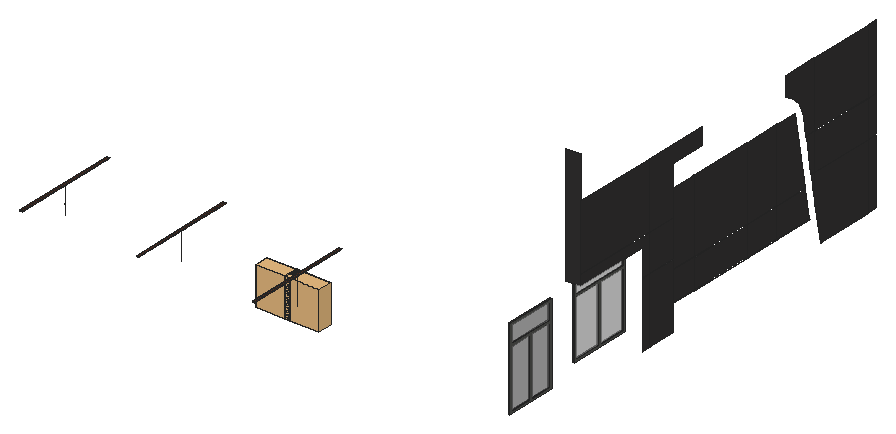
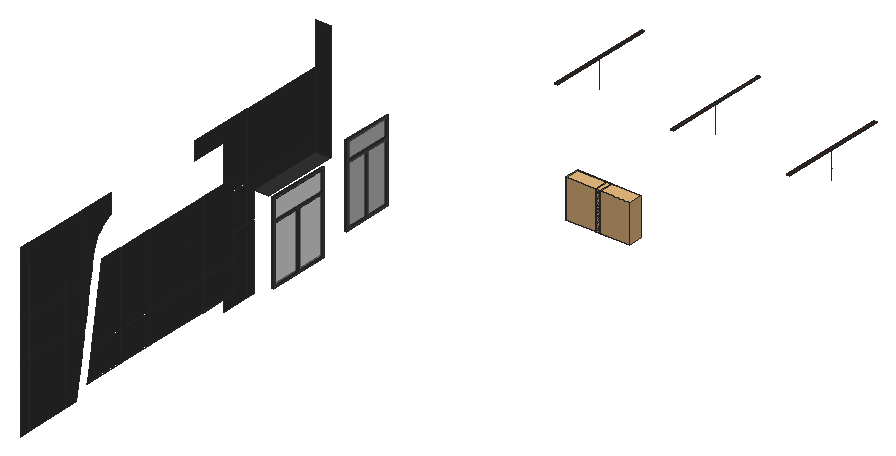
# SketchUp Ruby script. Lengths in inches.
U = 1.inch
M = Sketchup.active_model
def pt(a) = Geom::Point3d.new(a.map { |v| v * U })
def face(e, loops, mat)
  f = e.add_face(loops[0].map { |a| pt(a) })
  loops[1..].each { |l| e.add_face(l.map { |a| pt(a) }).erase! }
  f.material = f.back_material = mat if mat
  f
end
# faces: each face lists its corners as indices into pts; further lists are holes
def faces(e, pts, list, mat = nil) = list.each { |f| face(e, (f[0].is_a?(Array) ? f : [f]).map { |l| l.map { |i| pts[i] } }, mat) }
# xy, xz, yz: faces in a plane at the given z, y or x. An outline is a flat list of corners, or four numbers for a rectangle; further outlines are holes
def ring(l) = l.size == 4 ? [[l[0], l[1]], [l[2], l[1]], [l[2], l[3]], [l[0], l[3]]] : l.each_slice(2).to_a
def flat(e, list, mat, &to3) = list.each { |f| face(e, (f[0].is_a?(Array) ? f : [f]).map { |l| ring(l).map { |u, v| to3.(u, v) } }, mat) }
def xy(e, z, list, mat = nil) = flat(e, list, mat) { |x, y| [x, y, z] }
def xz(e, y, list, mat = nil) = flat(e, list, mat) { |x, z| [x, y, z] }
def yz(e, x, list, mat = nil) = flat(e, list, mat) { |y, z| [x, y, z] }
def lines(e, pts, list) = list.each { |a, b| e.add_line(pt(pts[a]), pt(pts[b])) }
# prism: a flat outline (further loops are holes) pulled along v
def prism(e, loops, v, mat = nil)
  f = face(e, loops, mat); d = Geom::Vector3d.new(v.map { |x| x * U })
  f.pushpull(f.normal.samedirection?(d) ? d.length : -d.length)
end
def box(e, o, s, mat = nil) = prism(e, [[o, [o[0] + s[0], o[1], o[2]], [o[0] + s[0], o[1] + s[1], o[2]], [o[0], o[1] + s[1], o[2]]]], [0, 0, s[2]], mat)
def at(x, y, z, deg = 0) = Geom::Transformation.translation(pt([x, y, z])) * Geom::Transformation.rotation(ORIGIN, Z_AXIS, deg.degrees)
def axes(o, x, y, z) = Geom::Transformation.new([*x, 0, *y, 0, *z, 0, *pt(o).to_a, 1])
def part(name) = M.definitions.add(name)
# library, detail: a bought-in or finely detailed component or shape, given as its bounding box
def library(name, o, s) = part(name).tap { |d| box(d.entities, o, s) }
def detail(e, o, s) = box(e.add_group.entities, o, s)
def put(e, d, t, mat = nil) = e.add_instance(d, t).tap { |i| i.material = mat if mat }
def group(e, t, mat = nil) = e.add_group.tap { |g| g.transformation = t; g.material = mat if mat }.entities
root = M.entities
M.materials.add("[Granite Dark Gray]").color = [51, 50, 50]
M.materials.add("[Metal Seamed]").color = [79, 80, 77]
M.materials.add("[Quartz Light Grey]").color = [251, 251, 252]
M.materials.add("[Translucent Glass Gray]").color = [183, 183, 183]
M.materials["[Translucent Glass Gray]"].alpha = 0.5
M.materials.add("[Translucent Glass Gray]2").color = [128, 128, 128]
M.materials["[Translucent Glass Gray]2"].alpha = 0.5
M.materials.add("[Wood Cherry Original]1").color = [93, 50, 33]
c1 = library("Wall Plant \#1",[1.06,-5.35,-7.67],[27.94,11.64,30.91])
c2 = part("Group1942\#1")
p = [[0,0,0],[0,0,-13.93],[-0.15,0,-13.93],[1,-44.1,0],[-1,-44.1,0],[1,44.1,0],
  [1,0,0],[-1,44.1,0],[0.15,0,-13.93],[-1,0,0],[0,0,-22.55]]
lines(c2.entities,p,[[0,1],[1,2],[3,4],[5,6],[7,5],[1,8],[9,0],[0,6],[8,10],[4,9],[6,3],[2,10],
  [9,7]])
c3 = part("Rectangle Light\#1")
put(c3.entities,c2,at(0,0,0))
c4 = part("12")
box(c4.entities,[0,0,-0.5],[2,125,0.5])
put(c4.entities,c3,axes([1,62.5,-0.51],[1,0,0],[0,1.41723,0],[0,0,1]))
xy(root,279,[[443.875,363,444,369],[443.875,370,444,393],[443.875,543.39,444,591],[443.875,592,444,600]],"[Granite Dark Gray]")
xy(root,294,[[436.875,393,437,423],[436.875,424,437,477],[436.875,478,437,507],[436.875,508,437,540.78]],"[Granite Dark Gray]")
xy(root,295,[[436.875,393,437,423],[436.875,424,437,477],[436.875,478,437,507],[436.875,508,437,540.61]],"[Granite Dark Gray]")
xy(root,318,[[436.875,423,437,424],[436.875,424,437,477],[436.875,478,437,507],[436.875,508,437,536.61]],"[Granite Dark Gray]")
xy(root,319,[[436.875,423,437,424],[436.875,424,437,477],[436.875,478,437,507],[436.875,508,437,536.43]],"[Granite Dark Gray]")
xy(root,332,[[443.875,363,444,369],[443.875,370,444,393],[443.875,534.17,444,537],[443.875,538,444,591],[443.875,592,444,600]],"[Granite Dark Gray]")
xy(root,333,[[443.875,363,444,369],[443.875,370,444,393],[443.875,534,444,537],[443.875,538,444,591],[443.875,592,444,600]],"[Granite Dark Gray]")
xy(root,354,[[432,300,444,363]],"[Granite Dark Gray]")
xy(root,362,[[443.875,300,444,369],[443.875,370,444,393],[443.875,528.96,444,537],[443.875,538,444,591],[443.875,592,444,600]],"[Granite Dark Gray]")
xy(root,363,[[443.875,300,444,369],[443.875,370,444,393],[443.875,528.78,444,537],[443.875,538,444,591],[443.875,592,444,600]],"[Granite Dark Gray]")
xz(root,300,[[432,354,444,354,444,362,443.875,362,443.875,363,444,363,444,416,443.875,416,443.875,417,444,417,444,450,432,450]],"[Granite Dark Gray]")
xz(root,369,[[443.875,279,444,332],[443.875,333,444,362],[443.875,363,444,416]],"[Granite Dark Gray]")
xz(root,370,[[443.875,279,444,332],[443.875,333,444,362],[443.875,363,444,416]],"[Granite Dark Gray]")
xz(root,423,[[436.875,295,437,318],[436.875,318,437,319],[436.875,319,437,378]],"[Granite Dark Gray]")
xz(root,424,[[436.875,295,437,318],[436.875,319,437,378]],"[Granite Dark Gray]")
xz(root,477,[[436.875,295,437,318],[436.875,319,437,378]],"[Granite Dark Gray]")
xz(root,478,[[436.875,295,437,318],[436.875,319,437,378]],"[Granite Dark Gray]")
xz(root,507,[[436.875,295,437,318],[436.875,319,437,378]],"[Granite Dark Gray]")
xz(root,508,[[436.875,295,437,318],[436.875,319,437,378]],"[Granite Dark Gray]")
xz(root,537,[[443.875,315.75,444,332],[443.875,333,444,362],[443.875,363,444,400.54]],"[Granite Dark Gray]")
xz(root,538,[[443.875,310,444,332],[443.875,333,444,362],[443.875,363,444,400.19]],"[Granite Dark Gray]")
xz(root,591,[[443.875,279,444,315.75],[443.875,315.75,444,332],[443.875,333,444,362],[443.875,363,444,400.54]],"[Granite Dark Gray]")
xz(root,592,[[443.875,279,444,310],[443.875,310,444,332],[443.875,333,444,362],[443.875,363,444,400.19]],"[Granite Dark Gray]")
yz(root,437,[[393,295,423,318],[424,295,477,318],[478,295,507,318],[508,295,540.61,295,536.61,318,508,318],[393,318,423,319],
  [393,319,423,378],[424,319,477,378],[478,319,507,378],[508,319,536.43,319,526.17,378,508,378]],"[Granite Dark Gray]")
yz(root,444,[[363,279,369,332],[370,279,393,332],[543.39,279,591,279,591,332,538,332,538,310],[592,279,600,332],[537,315.75,537,332,534.17,332],
  [363,333,369,333,369,362,300,362,300,354,363,354],[370,333,393,362],[534,333,537,333,537,362,528.96,362],[538,333,591,362],[592,333,600,362],
  [300,363,369,416],[370,363,393,363,393,402,423,402,423,416,370,416],[528.78,363,537,363,537,416,508,416,508,400.19,508.15,400.13,508.4,400.04,508.64,399.94,509.14,399.74,509.38,399.63,509.625,399.52,509.87,399.42,510.11,399.3,510.35,399.19,510.83,398.95,511.0625,398.83,511.3,398.71,511.53,398.59,511.77,398.46,512.23,398.2,512.46,398.0625,512.69,397.93,512.92,397.79,513.14,397.65,513.37,397.51,513.59,397.36,513.8125,397.22,514.03,397.07,514.47,396.77,514.6875,396.61,514.9,396.45,515.12,396.3,515.33,396.14,515.54,395.97,515.75,395.81,515.96,395.64,516.16,395.47,516.37,395.3,516.77,394.96,517.17,394.6,517.36,394.42,517.56,394.24,517.75,394.06,517.94,393.875,518.32,393.5,518.51,393.31,518.69,393.12,518.87,392.92,519.05,392.73,519.41,392.33,519.58,392.13,519.76,391.93,519.93,391.72,520.1,391.52,520.26,391.3125,520.43,391.1,521.07,390.26,521.23,390.04,521.83,389.16,521.97,388.9375,522.12,388.71,522.26,388.49,522.4,388.26,522.53,388.03,522.67,387.8,522.93,387.34,523.0625,387.11,523.3125,386.64,523.43,386.4,523.55,386.17,523.67,385.93,523.78,385.6875,523.9,385.45,524.01,385.2,524.12,384.96,524.22,384.72,524.33,384.47,524.43,384.23,524.53,383.98,524.72,383.48,524.8125,383.23,524.9,382.98,524.99,382.73,525.07,382.48,525.16,382.23,525.24,381.97,525.31,381.72,525.39,381.46,525.46,381.21,525.6,380.69,525.67,380.4375,525.73,380.18,525.91,379.4,525.96,379.14,526.02,378.88,526.07,378.62,526.11,378.35],[538,363,591,416],[592,363,600,416]],"[Granite Dark Gray]")
p = [[437,536.61,319],[437,536.43,319],[432,447,354],[432,447,355],[437,540.61,295],[437,540.78,295],
  [437,562,378],[437,562,319],[437,562,318],[437,562,295],[437,563,318],[437,563,295],
  [437,563,378],[437,563,319]]
lines(root,p,[[0,1],[2,3],[4,5],[6,7],[8,9],[10,11],[12,13]])
g1 = group(root,at(438,234,288),"[Quartz Light Grey]")
g2 = group(g1,at(0,0,0))
prism(g2,[[[0,42,66],[0,42,0],[0,0,0],[0,0,66]],[[0,20.25,1.5],[0,20.25,49],[0,1.5,49],[0,1.5,1.5]],[[0,21.75,1.5],[0,40.5,1.5],[0,40.5,49],[0,21.75,49]],[[0,40.5,50.5],[0,40.5,64.5],[0,1.5,64.5],[0,1.5,50.5]]],[1.5,0,0],"[Metal Seamed]")
g3 = group(g2,at(0.5,1.5,50.5),"[Translucent Glass Gray]2")
box(g3,[0,0,0],[0.47,39,14])
g4 = group(g2,at(0.5,21.75,1.5),"[Translucent Glass Gray]2")
box(g4,[0,0,0],[0.47,18.75,47.5])
g5 = group(g2,at(0.5,1.5,1.5),"[Translucent Glass Gray]2")
box(g5,[0,0,0],[0.47,18.75,47.5])
g6 = group(root,at(428,312,288),"[Quartz Light Grey]")
p = [[0,49.5,1.5],[0,49.5,47],[0,49.5,64.5],[0,1.5,64.5],[0,1.5,48.5],[0,1.5,1.5],
  [0,24.75,1.5],[0,49.5,48.5],[0,26.25,47],[0,1.5,47],[0,26.25,1.5],[0,24.75,47]]
lines(g6,p,[[0,1],[2,3],[3,4],[5,6],[7,4],[7,2],[1,8],[9,5],[8,10],[10,0],[11,6],[11,9]])
g7 = group(g6,at(0,0,0),"[Metal Seamed]")
prism(g7,[[[0,51,66],[0,51,0],[0,0,0],[0,0,66]],[[0,26.25,1.5],[0,49.5,1.5],[0,49.5,47],[0,26.25,47]],[[0,24.75,1.5],[0,24.75,47],[0,1.5,47],[0,1.5,1.5]],[[0,49.5,48.5],[0,49.5,64.5],[0,1.5,64.5],[0,1.5,48.5]]],[1.5,0,0])
g8 = group(g7,at(0.5,1.5,1.5),"[Translucent Glass Gray]")
box(g8,[0,24.75,0],[0.47,23.25,45.5])
box(g8,[0,0,47],[0.47,48,16])
box(g8,[0,0,0],[0.47,23.25,45.5])
put(root,c1,at(279.5,209.21,323.01),"[Quartz Light Grey]")
put(root,c1,at(255.5,209.21,323.01),"[Quartz Light Grey]")
put(root,c4,axes([336.25,101.3,392.75],[1,0,0],[0,0.7056,0],[0,0,1]),"[Wood Cherry Original]1")
put(root,c4,axes([242,101.3,392.75],[1,0,0],[0,0.7056,0],[0,0,1]),"[Wood Cherry Original]1")
put(root,c4,axes([147.75,101.3,392.75],[1,0,0],[0,0.7056,0],[0,0,1]),"[Wood Cherry Original]1")
